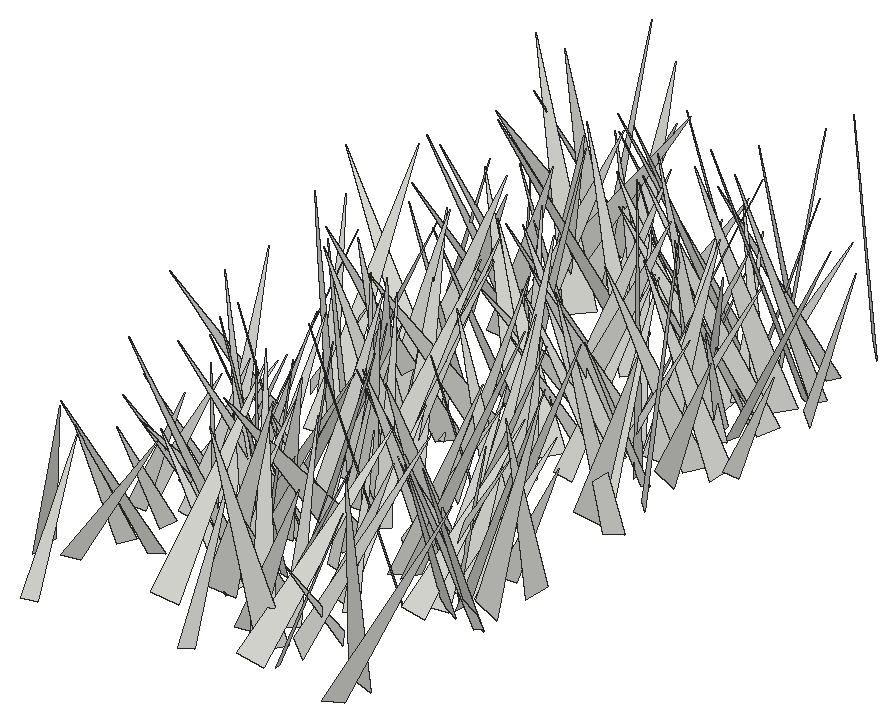
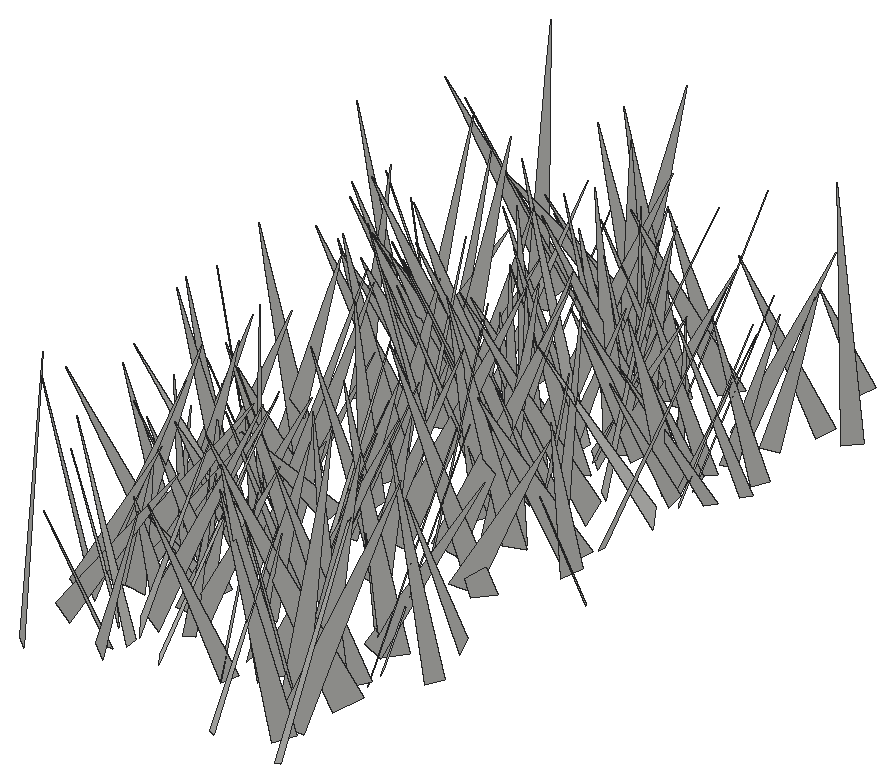
# SketchUp Ruby script. Lengths in inches.
U = 1.inch
M = Sketchup.active_model
def pt(a) = Geom::Point3d.new(a.map { |v| v * U })
def face(e, loops, mat)
  f = e.add_face(loops[0].map { |a| pt(a) })
  loops[1..].each { |l| e.add_face(l.map { |a| pt(a) }).erase! }
  f.material = f.back_material = mat if mat
  f
end
# faces: each face lists its corners as indices into pts; further lists are holes
def faces(e, pts, list, mat = nil) = list.each { |f| face(e, (f[0].is_a?(Array) ? f : [f]).map { |l| l.map { |i| pts[i] } }, mat) }
# xy, xz, yz: faces in a plane at the given z, y or x. An outline is a flat list of corners, or four numbers for a rectangle; further outlines are holes
def ring(l) = l.size == 4 ? [[l[0], l[1]], [l[2], l[1]], [l[2], l[3]], [l[0], l[3]]] : l.each_slice(2).to_a
def flat(e, list, mat, &to3) = list.each { |f| face(e, (f[0].is_a?(Array) ? f : [f]).map { |l| ring(l).map { |u, v| to3.(u, v) } }, mat) }
def xy(e, z, list, mat = nil) = flat(e, list, mat) { |x, y| [x, y, z] }
def xz(e, y, list, mat = nil) = flat(e, list, mat) { |x, z| [x, y, z] }
def yz(e, x, list, mat = nil) = flat(e, list, mat) { |y, z| [x, y, z] }
def lines(e, pts, list) = list.each { |a, b| e.add_line(pt(pts[a]), pt(pts[b])) }
# prism: a flat outline (further loops are holes) pulled along v
def prism(e, loops, v, mat = nil)
  f = face(e, loops, mat); d = Geom::Vector3d.new(v.map { |x| x * U })
  f.pushpull(f.normal.samedirection?(d) ? d.length : -d.length)
end
def box(e, o, s, mat = nil) = prism(e, [[o, [o[0] + s[0], o[1], o[2]], [o[0] + s[0], o[1] + s[1], o[2]], [o[0], o[1] + s[1], o[2]]]], [0, 0, s[2]], mat)
def at(x, y, z, deg = 0) = Geom::Transformation.translation(pt([x, y, z])) * Geom::Transformation.rotation(ORIGIN, Z_AXIS, deg.degrees)
def axes(o, x, y, z) = Geom::Transformation.new([*x, 0, *y, 0, *z, 0, *pt(o).to_a, 1])
def part(name) = M.definitions.add(name)
# library, detail: a bought-in or finely detailed component or shape, given as its bounding box
def library(name, o, s) = part(name).tap { |d| box(d.entities, o, s) }
def detail(e, o, s) = box(e.add_group.entities, o, s)
def put(e, d, t, mat = nil) = e.add_instance(d, t).tap { |i| i.material = mat if mat }
def group(e, t, mat = nil) = e.add_group.tap { |g| g.transformation = t; g.material = mat if mat }.entities
root = M.entities
c1 = part("fur_instance\#9")
p = [[0.8125,0,1.79],[0.67,-0.02,1.48],[0,-0.11,0],[0,0.11,0]]
faces(c1.entities,p,[[0,1,2,3]])
put(root,c1,axes([527.9,334.54,-21.66],[-5.38629,2.97439,0.98855],[2.72826,5.41671,-1.43257],[1.54299,0.80541,5.98388]))
put(root,c1,axes([528.33,331.44,-21.66],[-6.95908,-3.88864,0.42907],[-3.38575,6.42493,3.31533],[1.96017,-2.70799,7.24975]))
put(root,c1,axes([524.98,314.1875,-21.66],[6.92696,-1.79403,0.01467],[-1.72828,-6.68834,-1.86567],[-0.48147,-1.80253,6.90801]))
put(root,c1,axes([525.2,336.74,-21.66],[3.3764,2.66955,0.1135],[2.47122,-3.05035,-1.76859],[1.01611,-1.452,3.92412]))
put(root,c1,axes([528.0625,325.21,-21.66],[-4.13321,-3.41194,0.20507],[-3.07913,3.85633,2.10107],[1.48403,-1.5014,4.93054]))
put(root,c1,axes([531.46,339.43,-21.66],[-4.54084,5.90887,0.08971],[5.53212,4.21055,2.68494],[-2.07809,-1.7025,6.95162]))
put(root,c1,axes([528.06,317.37,-21.66],[2.83348,-4.00549,0.52306],[-3.76222,-2.8494,-1.43972],[-1.47079,-0.42795,4.69039]))
put(root,c1,axes([527.96,309.13,-21.66],[-3.50119,3.09472,0.56001],[2.74674,3.41714,-1.71109],[1.53177,0.94611,4.34831]))
put(root,c1,axes([527.43,344.36,-21.66],[5.0446,1.96996,1.21492],[1.59207,-5.06819,1.60732],[-1.6799,1.1124,5.17158]))
put(root,c1,axes([526.14,320.61,-21.66],[2.61538,-3.98544,0.72253],[-3.93735,-2.29982,1.56655],[0.95028,1.43982,4.50221]))
put(root,c1,axes([527.27,360.54,-21.66],[-5.00279,-6.48805,0.18943],[-5.66686,4.48249,3.86684],[3.16501,-2.22958,7.22289]))
put(root,c1,axes([528.46,323.44,-21.66],[-4.47086,-3.62986,0.22446],[-3.11938,4.01034,2.72058],[1.8697,-1.98902,5.07572]))
put(root,c1,axes([529.08,349.32,-21.66],[-5.93761,-4.29126,0.84113],[-3.95201,5.87307,2.0655],[1.8719,-1.21235,7.02879]))
put(root,c1,axes([525.89,322.12,-21.66],[1.52671,4.77623,1.67607],[4.63081,-0.61106,-2.47682],[2.04382,-2.18327,4.35989]))
put(root,c1,axes([529.09,357.24,-21.66],[4.10096,-6.21113,0.1393],[-5.64172,-3.79303,-3.03306],[-2.60165,-1.56533,6.79681]))
put(root,c1,axes([528.67,320.19,-21.66],[3.08843,-3.08617,0.55459],[-2.71507,-3.02147,-1.69397],[-1.56857,-0.84658,4.0241]))
put(root,c1,axes([528.79,350.86,-21.66],[-5.78164,-4.6449,0.78576],[-4.06196,5.54542,2.89287],[2.386,-1.8147,6.82889]))
put(root,c1,axes([528.7,333.09,-21.66],[-6.04626,5.73242,0.3376],[5.11125,5.59588,-3.47751],[2.61721,2.31459,7.57131]))
put(root,c1,axes([528.83,324.41,-21.66],[-4.31312,-2.31019,0.44376],[-1.59331,3.55068,2.99849],[1.73068,-2.4885,3.8664]))
put(root,c1,axes([530.14,317.34,-21.66],[-0.06223,-5.95217,0.13196],[-5.73579,0.02457,-1.59678],[-1.59576,0.14382,5.73432]))
put(root,c1,axes([530.96,347.81,-21.66],[-0.84326,-5.89202,0.02664],[-5.53518,0.78295,-2.04363],[-2.01949,0.3143,5.59022]))
put(root,c1,axes([529.37,323.89,-21.66],[-5.90287,3.96424,1.22936],[3.5461,5.92766,-2.08769],[2.15678,1.10365,6.7971]))
put(root,c1,axes([526.81,324,-21.66],[0.32449,4.79651,0.65441],[4.29347,0.01783,-2.25961],[2.23626,-0.73022,4.24334]))
put(root,c1,axes([528.8,322.51,-21.66],[3.99187,0.97882,1.10255],[0.50795,-3.90054,1.62373],[-1.38409,1.39155,3.77579]))
put(root,c1,axes([526.25,348.38,-21.66],[0.97454,-6.53217,0.4424],[-5.83998,-0.6651,3.04417],[2.95966,0.83851,5.86106]))
put(root,c1,axes([528.23,327.07,-21.66],[6.17595,4.1917,0.11311],[3.92557,-5.85042,2.46738],[-1.47413,1.98185,7.04448]))
put(root,c1,axes([528.51,324.95,-21.66],[4.2696,-0.12633,0.87704],[-0.45536,-4.01534,1.6384],[-0.76014,1.6958,3.94476]))
put(root,c1,axes([531.46,352.01,-21.66],[-4.16616,6.68617,2.08588],[7.00105,3.90518,1.46546],[-0.20279,-2.54114,7.74043]))
put(root,c1,axes([526.8,314.12,-21.66],[4.24231,-3.44067,0.07958],[-3.18347,-3.87509,2.16585],[1.3077,1.72835,5.01442]))
put(root,c1,axes([530.37,355.06,-21.66],[3.83849,6.3713,1.10198],[6.13828,-3.99344,1.70758],[-2.03209,-0.02789,7.23959]))
put(root,c1,axes([531.67,330.76,-21.66],[3.01287,6.59159,3.14785],[6.68601,-3.85992,1.68335],[-2.94198,-2.02171,7.04931]))
put(root,c1,axes([530.47,355.23,-21.66],[6.98287,-2.99298,2.96369],[-2.61118,-7.57832,-1.50091],[-3.30502,-0.33623,7.44753]))
put(root,c1,axes([531.56,346.69,-21.66],[2.74983,3.97442,1.3241],[3.39736,-3.04242,2.07665],[-2.45097,0.24187,4.36407]))
put(root,c1,axes([528.9,321.58,-21.66],[-0.2633,5.21725,2.01289],[5.21535,0.95622,-1.79623],[2.01778,-1.79073,4.90536]))
put(root,c1,axes([532.01,320.1,-21.66],[2.11114,4.26728,1.69749],[4.08085,-2.60007,1.46097],[-2.10662,-0.76029,4.53125]))
put(root,c1,axes([532.57,320.6,-21.66],[-6.5639,-4.29471,0.69968],[-4.06333,6.50273,1.7952],[1.55674,-1.13527,7.63588]))
put(root,c1,axes([533.91,329.45,-21.66],[-6.55777,-1.69063,0.96933],[-1.94723,5.82112,-3.02077],[0.07829,3.17151,6.06115]))
put(root,c1,axes([531.86,326.875,-21.66],[-4.79038,-5.44103,1.36632],[-5.2062,4.98101,1.5825],[2.08977,-0.06337,7.07448]))
put(root,c1,axes([529.21,351.17,-21.66],[3.36914,-5.54095,2.01408],[-5.73384,-2.5398,2.60427],[1.37175,2.99283,5.93894]))
put(root,c1,axes([534.72,324.05,-21.66],[-3.87014,-4.65436,0.40491],[-4.4497,3.51193,-2.16136],[-1.42379,1.67578,5.65416]))
put(root,c1,axes([529.17,352.91,-21.66],[-0.1774,-7.7519,1.13116],[-7.17611,0.61466,3.08685],[3.14245,0.96602,7.113]))
put(root,c1,axes([528.64,358.28,-21.66],[2.77166,-6.45652,0.14972],[-5.9267,-2.47813,2.8503],[2.56578,1.25036,6.42219]))
put(root,c1,axes([532.09,360.17,-21.66],[-3.9218,-4.42687,0.35438],[-4.07666,3.77609,2.05553],[1.7617,-1.11678,5.54549]))
put(root,c1,axes([534.25,352.14,-21.66],[-1.51333,-7.7582,0.0595],[-7.60064,1.47034,-1.59746],[-1.5568,0.36304,7.74132]))
put(root,c1,axes([531.94,321.66,-21.66],[6.07778,0.82962,2.17123],[-0.33597,-5.70106,3.1188],[-2.29992,3.02515,5.28212]))
put(root,c1,axes([531.69,331.08,-21.66],[4.95008,1.27612,1.12304],[0.89586,-4.89693,1.61571],[-1.4447,1.33589,4.84988]))
put(root,c1,axes([530.04,339.4,-21.66],[-0.29437,7.39176,2.68978],[7.28817,1.26884,-2.68928],[2.95898,-2.3899,6.89148]))
put(root,c1,axes([529.6875,347.4,-21.66],[2.97269,-7.01093,0.81561],[-6.80259,-2.60982,2.35986],[1.88234,1.64042,7.24024]))
put(root,c1,axes([535.32,319.31,-21.66],[0.70112,8.01126,1.73468],[7.49163,-1.33281,3.12731],[-3.32639,-1.31314,7.4089]))
put(root,c1,axes([534.71,336.81,-21.66],[1.87232,-8.06563,0.81969],[-7.60481,-2.03883,-2.69107],[-2.80947,0.14362,7.83059]))
put(root,c1,axes([528.28,353.23,-21.66],[5.80573,-6.03364,0.3689],[-5.4436,-4.99608,3.95649],[2.62833,2.98023,7.37953]))
put(root,c1,axes([534.64,324.07,-21.66],[-6.99156,-3.62516,0.34789],[-3.32905,6.6672,2.57109],[1.47657,-2.13338,7.444]))
put(root,c1,axes([532.94,322.17,-21.66],[-4.70627,4.28235,1.06672],[3.70191,4.67966,-2.45399],[2.40255,1.178,5.87073]))
put(root,c1,axes([531.13,328.6875,-21.66],[8.13391,1.72844,0.70897],[1.41113,-7.75982,2.72846],[-1.22428,2.53935,7.85515]))
put(root,c1,axes([533.78,333.8,-21.66],[-6.33507,2.2676,3.27677],[3.13305,6.63723,1.4641],[2.46237,-2.61105,6.56746]))
put(root,c1,axes([535.47,341.85,-21.66],[-2.86561,6.0597,1.12131],[6.09085,2.59686,1.53195],[-0.93747,-1.65086,6.5257]))
put(root,c1,axes([533.78,339.56,-21.66],[-6.24986,-4.52728,1.84324],[-4.17742,6.50052,1.80193],[2.5383,-0.44892,7.504]))
put(root,c1,axes([534.28,336.44,-21.66],[1.52611,3.71718,0.33458],[3.41655,-1.5369,1.49113],[-1.50217,0.28087,3.73135]))
put(root,c1,axes([535.61,352.125,-21.66],[-5.65883,0.17912,0.29432],[0.09895,5.4838,-1.43499],[0.33003,1.4272,5.47679]))
put(root,c1,axes([533.24,353.52,-21.66],[5.43285,-3.6045,3.64876],[-4.74936,-5.54221,1.59663],[-1.93634,3.48041,6.32132]))
put(root,c1,axes([532.07,334.23,-21.66],[0.54119,7.40359,2.44886],[7.61955,0.0202,-1.74498],[1.65906,-2.50787,7.21533]))
put(root,c1,axes([535.94,316.77,-21.66],[-4.58905,2.11277,0.48874],[2.15665,4.32669,1.54618],[-0.22698,-1.60562,4.80963]))
put(root,c1,axes([532.6,329.95,-21.66],[4.39475,-2.24157,1.41228],[-2.61052,-4.13054,1.56743],[-0.4521,2.06082,4.67778]))
put(root,c1,axes([532.31,334.05,-21.66],[1.32188,-7.44707,0.58602],[-7.30684,-1.16527,1.67389],[1.55318,0.85612,7.37593]))
put(root,c1,axes([536.4,331.47,-21.66],[1.94153,-7.03493,2.68991],[-6.84514,-2.80689,-2.40016],[-3.14163,1.7682,6.89195]))
put(root,c1,axes([536.97,319.77,-21.66],[-4.91979,-5.33902,1.78444],[-5.59743,4.38767,-2.30455],[-0.5985,2.85253,6.88466]))
put(root,c1,axes([537.23,345.11,-21.66],[-6.20853,-2.44848,0.56631],[-2.51301,6.03462,-1.45936],[-0.02325,1.56521,6.51238]))
put(root,c1,axes([533.54,313.79,-21.66],[-2.62249,6.7547,0.84995],[6.3246,2.75431,-2.37468],[2.5195,0.11678,6.84575]))
put(root,c1,axes([535.32,332.52,-21.66],[5.43527,-3.00495,4.38513],[-4.48513,-5.95873,1.47596],[-2.85354,3.64214,6.0327]))
put(root,c1,axes([535.88,325.4,-21.66],[2.95419,-3.46444,1.08183],[-2.95275,-3.10527,-1.88109],[-2.11044,-0.50488,4.14621]))
put(root,c1,axes([537.9375,348.4,-21.66],[-2.07893,6.71015,1.41675],[6.64432,1.60395,2.15305],[-1.69892,-1.93817,6.68674]))
put(root,c1,axes([535.4,355.3,-21.66],[-3.59225,-3.71334,1.0598],[-3.39845,3.72735,1.54069],[1.83374,-0.36648,4.93148]))
put(root,c1,axes([537.61,339.54,-21.66],[-2.28095,-6.51713,0.89519],[-6.46928,2.05047,-1.55597],[-1.19279,1.34151,6.72716]))
put(root,c1,axes([536.82,327.26,-21.66],[-6.72767,0.28008,1.7782],[-0.11729,6.79671,-1.51427],[1.7963,1.49276,6.56102]))
put(root,c1,axes([534.35,325.84,-21.66],[0.16131,6.95669,2.04491],[7.08472,0.28432,-1.5261],[1.54396,-2.03146,6.78915]))
put(root,c1,axes([537.33,337.95,-21.66],[4.76692,-6.38187,0.99404],[-5.33821,-4.5884,-3.85875],[-3.63592,-1.6304,6.96863]))
put(root,c1,axes([536.58,318.23,-21.66],[4.8815,3.3845,2.02519],[2.72156,-5.22275,2.16824],[-2.85471,0.80828,5.53015]))
put(root,c1,axes([535.3,348.37,-21.66],[-5.2335,-6.40482,0.23356],[-5.52847,4.66397,4.0186],[3.24225,-2.38569,7.22925]))
put(root,c1,axes([534.08,322.875,-21.66],[2.99312,-6.69994,0.30324],[-6.59145,-2.87731,1.48788],[1.23852,0.87852,7.18569]))
put(root,c1,axes([534.7,316.79,-21.66],[1.84734,5.85191,0.92453],[5.8229,-1.61485,-1.41361],[1.09242,-1.28828,5.97153]))
put(root,c1,axes([534.1,333.12,-21.66],[3.571,6.90444,0.98118],[6.89309,-3.32732,-1.67343],[1.05801,-1.62595,7.59098]))
put(root,c1,axes([536.84,344.78,-21.66],[-5.34969,-3.46152,0.37635],[-2.75195,4.62606,3.43064],[2.1332,-2.713,5.36954]))
put(root,c1,axes([533.3125,320.56,-21.66],[6.82569,-2.14516,0.01525],[-2.06759,-6.56497,1.95405],[0.57187,1.86856,6.88284]))
put(root,c1,axes([537.81,327.03,-21.66],[-6.09704,1.94582,1.05535],[1.61207,6.02238,-1.79053],[1.51697,1.42075,6.14444]))
put(root,c1,axes([538.27,316.05,-21.66],[-6.12572,-2.31991,2.2614],[-2.97153,5.95041,-1.94497],[1.2907,2.68904,6.25488]))
put(root,c1,axes([536.48,340.16,-21.66],[-7.17026,0.40545,3.85637],[-0.86926,7.73252,-2.42922],[3.77894,2.54801,6.75839]))
put(root,c1,axes([537.85,324.88,-21.66],[5.96387,-5.74764,0.45925],[-4.68382,-5.21453,-4.43673],[-3.36276,-2.93042,6.99418]))
put(root,c1,axes([539.97,339,-21.66],[-3.49983,5.63032,0.78088],[5.54982,3.18646,1.89866],[-1.22869,-1.64469,6.35172]))
put(root,c1,axes([535.53,347.51,-21.66],[2.61038,6.20008,1.07332],[6.21386,-2.35716,-1.49626],[0.99041,-1.55238,6.55868]))
put(root,c1,axes([534.82,329.92,-21.66],[4.52009,6.67395,0.30614],[6.59904,-4.40227,-1.46264],[1.04307,-1.07006,7.92676]))
put(root,c1,axes([539.29,355.69,-21.66],[-6.65977,-5.09555,0.25994],[-4.96209,6.56797,1.61994],[1.1874,-1.13219,8.22757]))
put(root,c1,axes([535.83,327.87,-21.66],[2.29516,-7.21123,1.1617],[-7.23425,-2.07612,1.40519],[1.00849,1.5189,7.43607]))
put(root,c1,axes([535,355,-21.66],[2.54302,-4.52945,1.06711],[-4.23804,-1.75205,2.66287],[1.92189,2.12978,4.46004]))
put(root,c1,axes([540.28,351.1875,-21.66],[-4.33976,4.07233,1.17149],[4.17045,3.80756,2.21352],[-0.75076,-2.38923,5.52429]))
put(root,c1,axes([538.4,322.1,-21.66],[3.46655,5.88623,0.70358],[5.62008,-3.5225,1.77941],[-1.8861,0.32244,6.59533]))
put(root,c1,axes([535.91,327.78,-21.66],[0.28527,8.21503,1.11931],[7.94931,0.04717,-2.37217],[2.35543,-1.15413,7.87026]))
put(root,c1,axes([537.84,310.27,-21.66],[4.12915,-1.39251,2.24683],[-2.1688,-4.1671,1.40312],[-1.51116,2.17563,4.12556]))
put(root,c1,axes([535.37,316.23,-21.66],[3.43501,-7.39782,1.03394],[-7.28345,-3.06455,2.27067],[1.65774,1.86463,7.83397]))
put(root,c1,axes([538.56,318.22,-21.66],[6.05789,3.57549,2.196],[3.19122,-6.43003,1.66595],[-2.72445,0.41853,6.83424]))
put(root,c1,axes([538.72,317.54,-21.66],[3.46816,-3.92613,0.03464],[-3.68547,-3.27126,-1.77763],[-1.35388,-1.15247,4.92774]))
put(root,c1,axes([535.99,323.51,-21.66],[7.97506,1.59703,0.67128],[1.71117,-7.75527,-1.87893],[-0.27022,-1.97686,7.91339]))
put(root,c1,axes([539.58,341.4,-21.66],[-4.13984,-2.04423,0.54277],[-1.65039,3.86825,1.98107],[1.32277,-1.57147,4.17043]))
put(root,c1,axes([541.1875,349.61,-21.66],[-1.53438,4.71255,0.03454],[4.47921,1.44703,1.55125],[-1.46492,-0.51147,4.70702]))
put(root,c1,axes([540.73,313.21,-21.66],[-0.59735,8.07244,1.41711],[8.08686,0.34954,1.4177],[-1.33238,-1.49761,7.96939]))
put(root,c1,axes([542.23,352.69,-21.66],[-3.30387,-7.05223,0.96215],[-6.92829,2.9435,-2.21582],[-1.63048,1.78244,7.4659]))
put(root,c1,axes([542.3,353.52,-21.66],[-6.0406,-4.0795,1.11122],[-4.22494,5.74856,-1.86274],[-0.16426,2.16279,7.04708]))
put(root,c1,axes([540.63,335.74,-21.66],[-7.20595,2.28011,2.02761],[1.9171,7.42879,-1.54068],[2.37378,0.922,7.39939]))
put(root,c1,axes([540.75,315.61,-21.66],[-5.40299,1.91129,1.15946],[1.49374,5.34299,-1.84687],[1.66317,1.41036,5.42535]))
put(root,c1,axes([539.65,352.65,-21.66],[4.21418,-1.38432,0.79636],[-0.98829,-4.02576,-1.76817],[-1.25452,-1.47878,4.06808]))
put(root,c1,axes([539.48,322.38,-21.66],[-1.38897,4.86037,0.26759],[4.61521,1.40338,-1.53442],[1.54748,0.17706,4.81643]))
put(root,c1,axes([537.22,345.25,-21.66],[1.67696,-6.87357,2.26471],[-6.67493,-0.57073,3.21041],[2.79647,2.7596,6.30488]))
put(root,c1,axes([543.72,321.36,-21.66],[-6.31099,-5.2237,1.0112],[-5.28027,5.95593,-2.18722],[-0.65451,2.31907,7.89505]))
put(root,c1,axes([542.36,356.98,-21.66],[-3.42492,-4.02626,1.68032],[-4.34426,2.9504,-1.78518],[-0.40205,2.41841,4.97534]))
put(root,c1,axes([541.5,313.11,-21.66],[3.93699,-6.31061,2.13001],[-6.14082,-4.39732,-1.67764],[-2.57895,0.83692,7.24632]))
put(root,c1,axes([541.54,327.08,-21.66],[4.33462,-5.23656,1.50263],[-4.77333,-4.57611,-2.17783],[-2.62578,-0.3257,6.43953]))
put(root,c1,axes([538.33,332.48,-21.66],[4.58596,6.39713,1.96066],[6.63658,-4.04695,-2.31874],[0.85046,-2.91504,7.52182]))
put(root,c1,axes([541.64,350.63,-21.66],[1.73038,-3.85975,0.19684],[-3.59553,-1.68683,-1.46882],[-1.41726,-0.43309,3.96667]))
put(root,c1,axes([544.07,325.21,-21.66],[-4.22462,-4.77942,0.40733],[-4.62488,3.91455,-2.0354],[-1.27248,1.63999,6.04544]))
put(root,c1,axes([542.27,318.82,-21.66],[-4.53148,2.02632,0.31118],[1.79338,4.28391,-1.78018],[0.99329,1.50971,4.63371]))
put(root,c1,axes([543.11,340.1,-21.66],[-6.87965,3.10007,2.46286],[3.78941,6.58637,2.29475],[1.14737,-3.16466,7.18848]))
put(root,c1,axes([541.08,331.48,-21.66],[-4.09949,-5.26965,1.04192],[-4.89422,4.20438,2.00758],[2.21389,-0.46331,6.36747]))
put(root,c1,axes([543,330.99,-21.66],[1.40362,-5.52471,3.15038],[-5.88186,-2.35471,-1.50878],[-2.41887,2.51999,5.49692]))
put(root,c1,axes([543.6,339.36,-21.66],[-5.93019,0.58333,0.46706],[0.68124,5.75556,1.46115],[0.30714,-1.50292,5.77689]))
put(root,c1,axes([543.97,349.59,-21.66],[-6.77007,0.71674,0.61078],[0.8862,6.3486,2.37288],[0.31848,-2.42944,6.38099]))
put(root,c1,axes([542.75,342.65,-21.66],[-5.36407,2.31527,0.60969],[2.0889,5.25672,-1.5839],[1.1699,1.22955,5.6236]))
put(root,c1,axes([541.87,337.48,-21.66],[-5.06896,3.36354,0.19703],[2.56301,4.08037,-3.71862],[2.18706,3.01393,4.81452]))
put(root,c1,axes([542.17,343.04,-21.66],[-7.59167,-1.95799,2.55179],[-0.44126,7.11339,4.14535],[3.18601,-3.68034,6.65457]))
put(root,c1,axes([539.23,313.8125,-21.66],[3.81645,-5.44593,0.15233],[-5.28758,-3.65777,1.70554],[1.31259,1.09964,6.42764]))
put(root,c1,axes([540.49,312.93,-21.66],[5.57667,1.59527,0.3002],[1.43066,-5.3377,1.78788],[-0.76695,1.64269,5.51794]))
put(root,c1,axes([541.35,349.5,-21.66],[5.83634,-0.86723,1.56304],[-0.35494,-5.79341,-1.88904],[-1.75191,-1.71533,5.58985]))
put(root,c1,axes([542.1,347.72,-21.66],[3.66299,2.22216,0.32756],[1.7102,-3.16536,2.34915],[-1.4562,1.87225,3.58288]))
put(root,c1,axes([541.68,332.14,-21.66],[6.54564,-3.57049,3.76512],[-4.66006,-6.71077,1.73761],[-2.28219,3.46223,7.25083]))
put(root,c1,axes([540.63,319.49,-21.66],[1.73127,-4.9492,1.56465],[-4.93445,-1.0575,2.11492],[1.61056,2.08017,4.79781]))
put(root,c1,axes([547.43,348.13,-21.66],[-2.51256,7.06983,2.10699],[6.38069,0.96553,4.36915],[-3.70253,-3.13371,6.09968]))
put(root,c1,axes([541.33,311.36,-21.66],[-3.48939,6.7058,0.49493],[5.71017,3.24965,-3.77124],[3.55058,1.36403,6.55144]))
put(root,c1,axes([546.32,348.29,-21.66],[-2.71557,-5.16024,0.69315],[-4.67023,2.06855,-2.89705],[-2.30163,1.89099,5.06058]))
put(root,c1,axes([540.08,326.11,-21.66],[4.10846,4.74791,0.21399],[4.46685,-3.7608,-2.31765],[1.62348,-1.66782,5.83529]))
put(root,c1,axes([546.54,354.86,-21.66],[-1.84266,-5.86998,0.99209],[-5.21002,1.08759,-3.24178],[-2.88039,1.78795,5.22904]))
put(root,c1,axes([541.13,348.04,-21.66],[5.01849,-2.22986,0.6447],[-2.32023,-4.77497,1.54574],[0.06662,1.67347,5.26955]))
put(root,c1,axes([544.16,349.6875,-21.66],[-4.2837,1.86088,0.37109],[1.60299,4.03921,-1.75094],[1.01537,1.47394,4.32979]))
put(root,c1,axes([545.87,345.51,-21.66],[-0.49595,7.7495,2.67586],[7.77568,-0.40515,2.61451],[-2.59882,-2.6911,7.31198]))
put(root,c1,axes([544.89,340.14,-21.66],[-7.31055,-2.64435,2.80127],[-3.45475,7.15889,-2.25809],[1.70424,3.16886,7.43894]))
put(root,c1,axes([545.06,350.5,-21.66],[-1.00856,5.27208,0.80529],[5.17147,0.76643,1.45913],[-1.30357,-1.0384,5.16556]))
put(root,c1,axes([544.01,342.75,-21.66],[-5.33853,3.8285,0.2094],[3.37353,4.86067,-2.86257],[1.82225,2.21756,5.91295]))
put(root,c1,axes([542.89,311.82,-21.66],[4.06306,2.1594,0.43468],[1.91332,-3.91175,1.54848],[-1.0914,1.18135,4.33286]))
put(root,c1,axes([543.93,353.44,-21.66],[4.5947,4.98178,1.41698],[4.55399,-4.78808,2.06705],[-2.46722,0.43974,6.4542]))
put(root,c1,axes([542.96,326.35,-21.66],[6.488,-4.94571,0.82766],[-4.48999,-6.33233,-2.64212],[-2.23271,-1.63731,7.71838]))
put(root,c1,axes([541.55,344.0625,-21.66],[7.40987,3.38689,0.1989],[3.26816,-7.25381,1.76579],[-0.91088,1.52574,7.95356]))
put(root,c1,axes([543.72,316.36,-21.66],[-3.33896,-2.6162,0.26799],[-2.1089,2.92233,2.25332],[1.57125,-1.6372,3.59384]))
put(root,c1,axes([541.6875,323.76,-21.66],[6.12264,-2.56902,1.18593],[-2.80714,-5.86992,1.77677],[-0.35534,2.10644,6.39763]))
put(root,c1,axes([541.58,355.21,-21.66],[6.21728,1.67139,0.47713],[1.73743,-6.02723,-1.52629],[-0.05031,-1.59834,6.25448]))
put(root,c1,axes([545.96,339.4375,-21.66],[-1.77005,-3.87903,0.89181],[-3.77258,1.32393,-1.7292],[-1.26879,1.475,3.89741]))
put(root,c1,axes([544.72,325.9,-21.66],[-4.05266,-1.43323,0.72397],[-1.06557,3.87082,1.69814],[1.20119,-1.40176,3.94899]))
put(root,c1,axes([542.14,356.3125,-21.66],[2.38056,3.51502,0.37387],[3.33138,-2.08023,-1.65431],[1.18197,-1.21634,3.90969]))
put(root,c1,axes([546.88,352.03,-21.66],[-4.74845,-6.02691,1.04144],[-6.05438,4.44477,-1.88271],[-0.8676,1.96887,7.4382]))
put(root,c1,axes([547.53,352.37,-21.66],[-2.26256,-5.81888,2.33683],[-5.71547,0.89178,-3.31322],[-2.57945,3.12805,5.2916]))
put(root,c1,axes([544.95,324.96,-21.66],[-6.41092,4.00729,0.82453],[3.32918,6.00061,-3.27831],[2.37798,2.40258,6.81256]))
put(root,c1,axes([542.39,349.19,-21.66],[6.00758,0.21792,0.49644],[0.387,-5.59183,-2.22857],[-0.3797,-2.2514,5.58318]))
put(root,c1,axes([546.59,350.43,-21.66],[2.25381,-7.00366,2.80187],[-6.80723,-3.14832,-2.39397],[-3.25014,1.7373,6.957]))
put(root,c1,axes([542.36,323.92,-21.66],[8.0865,0.10169,1.15451],[-0.2162,-7.86244,2.20681],[-1.13864,2.21504,7.78021]))
put(root,c1,axes([545.6,336.13,-21.66],[-5.23053,3.77379,0.03544],[3.44734,4.80229,-2.57973],[1.53577,2.07308,5.91142]))
put(root,c1,axes([542.67,346.74,-21.66],[3.6305,3.98779,0.322],[3.84064,-3.3521,-1.78874],[1.12055,-1.43096,5.08758]))
put(root,c1,axes([546.9375,342.54,-21.66],[2.35436,-6.19743,2.05043],[-5.78585,-2.99044,-2.39512],[-3.02263,0.89697,6.18179]))
put(root,c1,axes([545.66,321.93,-21.66],[-4.8564,4.18897,0.42907],[3.70643,4.56321,-2.59917],[1.99849,1.71635,5.86314]))
put(root,c1,axes([543.1,340.43,-21.66],[3.75203,3.55416,0.24846],[3.4305,-3.50645,-1.64561],[0.96201,-1.35805,4.89916]))
put(root,c1,axes([548.77,321.62,-21.66],[-3.53185,-5.19128,1.06072],[-4.89285,2.7062,-3.04713],[-2.03336,2.50511,5.48984]))
put(root,c1,axes([542.59,313.93,-21.66],[4.68977,6.59581,0.10077],[6.41242,-4.52929,-1.96857],[1.54784,-1.22048,7.85006]))
put(root,c1,axes([544.22,324.07,-21.66],[7.47336,0.82298,1.26079],[0.38429,-7.21504,2.43175],[-1.45575,2.3203,7.11442]))
put(root,c1,axes([547.96,334.25,-21.66],[-0.65544,-6.57541,2.82853],[-6.91722,-0.14862,-1.94837],[-1.84083,2.89967,6.31422]))
put(root,c1,axes([545.5,346.6,-21.66],[4.05773,-0.76512,0.97615],[-0.40955,-3.97873,-1.41614],[-1.1707,-1.26007,3.87881]))
put(root,c1,axes([544.7,342.02,-21.66],[3.44666,-5.98968,2.82803],[-6.61551,-2.95389,1.80641],[0.33028,3.33943,6.67028]))
put(root,c1,axes([544.87,327.4,-21.66],[6.92746,0.46404,1.30725],[0.06508,-6.75935,2.05449],[-1.38564,2.00246,6.63205]))
put(root,c1,axes([544.94,320.84,-21.66],[-2.23637,5.81255,0.47787],[5.16217,2.21098,-2.73477],[2.71405,0.58421,5.59536]))
put(root,c1,axes([548.34,342.92,-21.66],[-6.51837,1.52305,1.37348],[1.82295,6.39951,1.5551],[0.93967,-1.84981,6.5108]))
put(root,c1,axes([546.23,358.75,-21.66],[-5.2101,-5.93708,2.74108],[-5.84341,5.80017,1.45611],[2.93548,1.00834,7.76362]))
put(root,c1,axes([546.29,322.21,-21.66],[-1.98153,-6.18192,0.39554],[-6.00617,2.01899,1.46585],[1.5161,-0.08133,6.32408]))
put(root,c1,axes([545.38,324.1,-21.66],[4.29125,3.34973,1.68987],[3.74545,-3.97458,-1.63261],[-0.21889,-2.33948,5.19327]))
put(root,c1,axes([543.3125,324.0625,-21.66],[5.8756,3.65861,0.2575],[3.32747,-5.11292,-3.2803],[1.54262,-2.90637,6.0949]))
put(root,c1,axes([547.3125,337.59,-21.66],[5.31201,5.41879,2.20999],[5.24419,-5.73235,1.45032],[-2.59727,-0.49162,7.44831]))
put(root,c1,axes([545.86,323.89,-21.66],[-0.77489,5.32124,0.74593],[4.8544,1.01638,-2.20776],[2.30365,-0.35187,4.90325]))
put(root,c1,axes([546.62,323.01,-21.66],[6.71372,1.26121,1.18447],[0.98901,-6.69183,1.51954],[-1.41968,1.3025,6.66001]))
put(root,c1,axes([545.71,334.73,-21.66],[2.64878,-6.42579,1.07864],[-6.29914,-2.22772,2.19734],[1.66585,1.79353,6.59382]))
put(root,c1,axes([546.38,346.33,-21.66],[6.37696,0.70596,0.43543],[0.57496,-6.19552,1.62437],[-0.59783,1.57187,6.20688]))
put(root,c1,axes([547.55,313.01,-21.66],[-1.05079,-7.8114,1.55453],[-7.7743,1.34665,1.51176],[1.73053,1.30661,7.73542]))
put(root,c1,axes([546.52,326.88,-21.66],[2.75762,-4.13306,0.47465],[-3.98702,-2.46295,1.71739],[1.18791,1.32801,4.66232]))
put(root,c1,axes([548.21,322.12,-21.66],[-2.24137,-6.8028,0.2078],[-6.58087,2.22202,1.76064],[1.73594,-0.35988,6.94277]))
put(root,c1,axes([548.78,326.64,-21.66],[5.89812,-2.41371,1.85981],[-1.99813,-6.12286,-1.60962],[-2.30052,-0.87028,6.16628]))
put(root,c1,axes([546.375,340.58,-21.66],[0.60809,-6.43634,0.77652],[-5.71222,-0.16309,3.1214],[3.06594,0.97271,5.66154]))
put(root,c1,axes([548.17,350.52,-21.66],[3.55889,4.26793,1.49162],[4.48448,-3.09137,-1.85436],[0.57409,-2.30955,5.23854]))
put(root,c1,axes([547.84,323.48,-21.66],[2.12208,6.92928,3.4126],[7.54208,-1.09525,-2.46604],[1.66665,-3.86645,6.81445]))
put(root,c1,axes([547.625,310.62,-21.66],[6.83257,-2.01041,0.78824],[-2.1593,-6.33413,2.56189],[0.022,2.68032,6.64549]))
put(root,c1,axes([548.81,343.22,-21.66],[2.19638,-3.75423,0.49776],[-3.62923,-1.92217,1.51658],[1.08198,1.1735,4.07656]))
